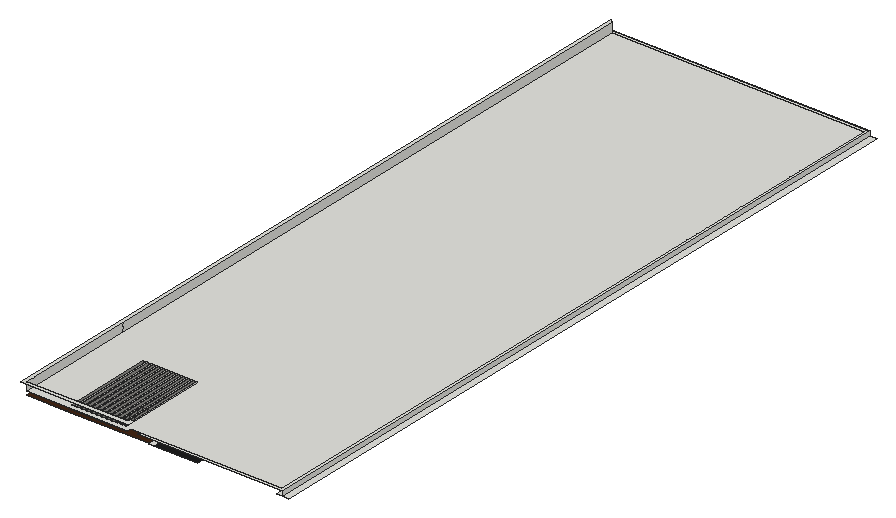
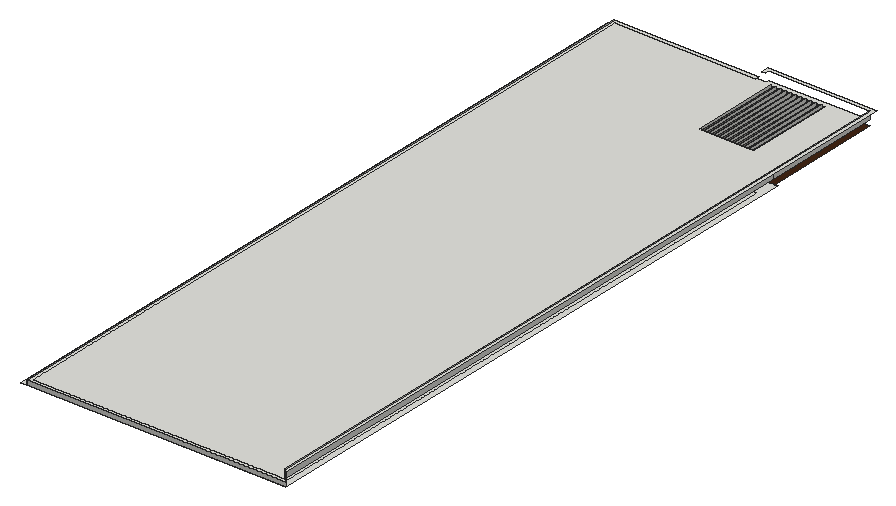
# SketchUp Ruby script. Lengths in inches.
U = 1.inch
M = Sketchup.active_model
def pt(a) = Geom::Point3d.new(a.map { |v| v * U })
def face(e, loops, mat)
  f = e.add_face(loops[0].map { |a| pt(a) })
  loops[1..].each { |l| e.add_face(l.map { |a| pt(a) }).erase! }
  f.material = f.back_material = mat if mat
  f
end
# faces: each face lists its corners as indices into pts; further lists are holes
def faces(e, pts, list, mat = nil) = list.each { |f| face(e, (f[0].is_a?(Array) ? f : [f]).map { |l| l.map { |i| pts[i] } }, mat) }
# xy, xz, yz: faces in a plane at the given z, y or x. An outline is a flat list of corners, or four numbers for a rectangle; further outlines are holes
def ring(l) = l.size == 4 ? [[l[0], l[1]], [l[2], l[1]], [l[2], l[3]], [l[0], l[3]]] : l.each_slice(2).to_a
def flat(e, list, mat, &to3) = list.each { |f| face(e, (f[0].is_a?(Array) ? f : [f]).map { |l| ring(l).map { |u, v| to3.(u, v) } }, mat) }
def xy(e, z, list, mat = nil) = flat(e, list, mat) { |x, y| [x, y, z] }
def xz(e, y, list, mat = nil) = flat(e, list, mat) { |x, z| [x, y, z] }
def yz(e, x, list, mat = nil) = flat(e, list, mat) { |y, z| [x, y, z] }
def lines(e, pts, list) = list.each { |a, b| e.add_line(pt(pts[a]), pt(pts[b])) }
# prism: a flat outline (further loops are holes) pulled along v
def prism(e, loops, v, mat = nil)
  f = face(e, loops, mat); d = Geom::Vector3d.new(v.map { |x| x * U })
  f.pushpull(f.normal.samedirection?(d) ? d.length : -d.length)
end
def box(e, o, s, mat = nil) = prism(e, [[o, [o[0] + s[0], o[1], o[2]], [o[0] + s[0], o[1] + s[1], o[2]], [o[0], o[1] + s[1], o[2]]]], [0, 0, s[2]], mat)
def at(x, y, z, deg = 0) = Geom::Transformation.translation(pt([x, y, z])) * Geom::Transformation.rotation(ORIGIN, Z_AXIS, deg.degrees)
def axes(o, x, y, z) = Geom::Transformation.new([*x, 0, *y, 0, *z, 0, *pt(o).to_a, 1])
def part(name) = M.definitions.add(name)
# library, detail: a bought-in or finely detailed component or shape, given as its bounding box
def library(name, o, s) = part(name).tap { |d| box(d.entities, o, s) }
def detail(e, o, s) = box(e.add_group.entities, o, s)
def put(e, d, t, mat = nil) = e.add_instance(d, t).tap { |i| i.material = mat if mat }
def group(e, t, mat = nil) = e.add_group.tap { |g| g.transformation = t; g.material = mat if mat }.entities
root = M.entities
M.materials.add("[Color M08]").color = [30, 30, 30]
M.materials.add("[Field Square Tile]").color = [211, 167, 108]
M.materials.add("[Granite Light Gray]").color = [149, 148, 144]
M.materials.add("[Wood Veneer 01]").color = [66, 38, 20]
xy(root,380.5,[[1555.29,511.08,1555.29,1825.82,1107.53,1825.82,1107.53,762.17,1323.53,762.17,1323.53,727.2,1097.72,727.2,1097.72,1835.625,1565.1,1835.625,1565.1,511.08],[1323.53,511.08,1332.45,589.83],[1565.1,511.08,1576.91,1835.625],[1323.53,589.83,1323.53,762.17,1107.53,762.17,1107.53,1825.82,1555.29,1825.82,1555.29,589.83,1508.52,589.83,1508.52,697.21,1413.21,697.21,1413.21,738.02,1332.45,738.02,1332.45,697.21,1323.83,697.21,1323.83,589.83],[1323.83,589.83,1332.45,697.21],
  [1413.21,589.83,1508.52,697.21],[1332.45,697.21,1413.21,738.02]])
xy(root,380.5,[[1332.45,511.08,1413.21,697.21]],"[Color M08]")
xy(root,380.5,[[[1102.55,512.27,1174.48,727.2],[1119.58,606.01,1121.1,606.38,1122.48,607.14,1123.61,608.22,1124.42,609.56,1124.85,611.0625,1124.89,612.63,1124.51,614.15,1123.76,615.52,1122.67,616.65,1121.33,617.46,1119.83,617.9,1118.26,617.93,1116.74,617.56,1115.37,616.81,1114.24,615.72,1113.43,614.38,1112.99,612.875,1112.96,611.3125,1113.33,609.79,1114.09,608.42,1115.17,607.29,1116.51,606.48,1118.02,606.04],[1119.58,554.26,1121.1,554.63,1122.48,555.39,1123.61,556.47,1124.42,557.81,1124.85,559.3125,1124.89,560.88,1124.51,562.4,1123.76,563.77,1122.67,564.9,1121.33,565.71,1119.83,566.15,1118.26,566.18,1116.74,565.81,1115.37,565.06,1114.24,563.97,1113.43,562.63,1112.99,561.125,1112.96,559.5625,1113.33,558.04,1114.09,556.67,1115.17,555.54,1116.51,554.73,1118.02,554.29],[1119.58,523.51,1121.1,523.88,1122.48,524.64,1123.61,525.72,1124.42,527.06,1124.85,528.5625,1124.89,530.13,1124.51,531.65,1123.76,533.02,1122.67,534.15,1121.33,534.96,1119.83,535.4,1118.26,535.43,1116.74,535.06,1115.37,534.31,1114.24,533.22,1113.43,531.88,1112.99,530.375,1112.96,528.8125,1113.33,527.29,1114.09,525.92,1115.17,524.79,1116.51,523.98,1118.02,523.54],[1119.58,666.01,1121.1,666.38,1122.48,667.14,1123.61,668.22,1124.42,669.56,1124.85,671.0625,1124.89,672.63,1124.51,674.15,1123.76,675.52,1122.67,676.65,1121.33,677.46,1119.83,677.9,1118.26,677.93,1116.74,677.56,1115.37,676.81,1114.24,675.72,1113.43,674.38,1112.99,672.875,1112.96,671.3125,1113.33,669.79,1114.09,668.42,1115.17,667.29,1116.51,666.48,1118.02,666.04],[1159.33,606.01,1160.85,606.38,1162.23,607.14,1163.36,608.22,1164.17,609.56,1164.6,611.0625,1164.64,612.63,1164.26,614.15,1163.51,615.52,1162.42,616.65,1161.08,617.46,1159.58,617.9,1158.01,617.93,1156.49,617.56,1155.12,616.81,1153.99,615.72,1153.18,614.38,1152.74,612.875,1152.71,611.3125,1153.08,609.79,1153.84,608.42,1154.92,607.29,1156.26,606.48,1157.77,606.04],[1159.33,554.26,1160.85,554.63,1162.23,555.39,1163.36,556.47,1164.17,557.81,1164.6,559.3125,1164.64,560.88,1164.26,562.4,1163.51,563.77,1162.42,564.9,1161.08,565.71,1159.58,566.15,1158.01,566.18,1156.49,565.81,1155.12,565.06,1153.99,563.97,1153.18,562.63,1152.74,561.125,1152.71,559.5625,1153.08,558.04,1153.84,556.67,1154.92,555.54,1156.26,554.73,1157.77,554.29],[1159.33,523.51,1160.85,523.88,1162.23,524.64,1163.36,525.72,1164.17,527.06,1164.6,528.5625,1164.64,530.13,1164.26,531.65,1163.51,533.02,1162.42,534.15,1161.08,534.96,1159.58,535.4,1158.01,535.43,1156.49,535.06,1155.12,534.31,1153.99,533.22,1153.18,531.88,1152.74,530.375,1152.71,528.8125,1153.08,527.29,1153.84,525.92,1154.92,524.79,1156.26,523.98,1157.77,523.54],[1159.33,666.01,1160.85,666.38,1162.23,667.14,1163.36,668.22,1164.17,669.56,1164.6,671.0625,1164.64,672.63,1164.26,674.15,1163.51,675.52,1162.42,676.65,1161.08,677.46,1159.58,677.9,1158.01,677.93,1156.49,677.56,1155.12,676.81,1153.99,675.72,1153.18,674.38,1152.74,672.875,1152.71,671.3125,1153.08,669.79,1153.84,668.42,1154.92,667.29,1156.26,666.48,1157.77,666.04]],[[1174.48,512.27,1323.53,727.2],[1269.93,519.43,1276.18,680.49],[1260.81,519.43,1267.06,680.49],[1251.68,519.43,1257.93,680.49],[1242.56,519.43,1248.81,680.49],[1233.43,519.43,1239.68,680.49],[1224.31,519.43,1230.56,680.49],[1215.18,519.43,1221.43,680.49],[1206.06,519.43,1212.31,680.49],[1196.93,519.43,1203.18,680.49],[1187.81,519.43,1194.06,680.49],[1178.68,519.43,1184.93,680.49]]],"[Wood Veneer 01]")
xy(root,381.875,[[1119.58,554.26,1118.02,554.29,1116.51,554.73,1115.17,555.54,1114.09,556.67,1113.33,558.04,1112.96,559.5625,1112.99,561.125,1113.43,562.63,1114.24,563.97,1115.37,565.06,1116.74,565.81,1118.26,566.18,1119.83,566.15,1121.33,565.71,1122.67,564.9,1123.76,563.77,1124.51,562.4,1124.89,560.88,1124.85,559.3125,1124.42,557.81,1123.61,556.47,1122.48,555.39,1121.1,554.63],[1159.33,554.26,1157.77,554.29,1156.26,554.73,1154.92,555.54,1153.84,556.67,1153.08,558.04,1152.71,559.5625,1152.74,561.125,1153.18,562.63,1153.99,563.97,1155.12,565.06,1156.49,565.81,1158.01,566.18,1159.58,566.15,1161.08,565.71,1162.42,564.9,1163.51,563.77,1164.26,562.4,1164.64,560.88,1164.6,559.3125,1164.17,557.81,1163.36,556.47,1162.23,555.39,1160.85,554.63],[1119.58,606.01,1118.02,606.04,1116.51,606.48,1115.17,607.29,1114.09,608.42,1113.33,609.79,1112.96,611.3125,1112.99,612.875,1113.43,614.38,1114.24,615.72,1115.37,616.81,1116.74,617.56,1118.26,617.93,1119.83,617.9,1121.33,617.46,1122.67,616.65,1123.76,615.52,1124.51,614.15,1124.89,612.63,1124.85,611.0625,1124.42,609.56,1123.61,608.22,1122.48,607.14,1121.1,606.38],[1159.33,606.01,1157.77,606.04,1156.26,606.48,1154.92,607.29,1153.84,608.42,1153.08,609.79,1152.71,611.3125,1152.74,612.875,1153.18,614.38,1153.99,615.72,1155.12,616.81,1156.49,617.56,1158.01,617.93,1159.58,617.9,1161.08,617.46,1162.42,616.65,1163.51,615.52,1164.26,614.15,1164.64,612.63,1164.6,611.0625,1164.17,609.56,1163.36,608.22,1162.23,607.14,1160.85,606.38],[1119.58,666.01,1118.02,666.04,1116.51,666.48,1115.17,667.29,1114.09,668.42,1113.33,669.79,1112.96,671.3125,1112.99,672.875,1113.43,674.38,1114.24,675.72,1115.37,676.81,1116.74,677.56,1118.26,677.93,1119.83,677.9,1121.33,677.46,1122.67,676.65,1123.76,675.52,1124.51,674.15,1124.89,672.63,1124.85,671.0625,1124.42,669.56,1123.61,668.22,1122.48,667.14,1121.1,666.38],
  [1159.33,666.01,1157.77,666.04,1156.26,666.48,1154.92,667.29,1153.84,668.42,1153.08,669.79,1152.71,671.3125,1152.74,672.875,1153.18,674.38,1153.99,675.72,1155.12,676.81,1156.49,677.56,1158.01,677.93,1159.58,677.9,1161.08,677.46,1162.42,676.65,1163.51,675.52,1164.26,674.15,1164.64,672.63,1164.6,671.0625,1164.17,669.56,1163.36,668.22,1162.23,667.14,1160.85,666.38]],"[Field Square Tile]")
xy(root,388.625,[[[1104.06,510.87,1287.38,510.87,1287.38,517.43,1558.75,517.43,1558.75,1829.28,1104.06,1829.28],[1178.68,519.43,1184.93,680.49],[1187.81,519.43,1194.06,680.49],[1196.93,519.43,1203.18,680.49],[1206.06,519.43,1212.31,680.49],[1215.18,519.43,1221.43,680.49],[1224.31,519.43,1230.56,680.49],[1233.43,519.43,1239.68,680.49],[1242.56,519.43,1248.81,680.49],[1251.68,519.43,1257.93,680.49],[1260.81,519.43,1267.06,680.49],[1269.93,519.43,1276.18,680.49]],[1304.4375,511.08,1565.1,511.08,1565.1,1835.625,1097.72,1835.625,1104.06,1829.28,1558.75,1829.28,1558.75,517.43,1304.4375,517.43]])
xy(root,403.8125,[[1097.72,504.52,1293.73,504.52,1293.73,517.43,1287.38,517.43,1287.38,510.87,1104.06,510.87,1104.06,1829.28,1097.72,1835.625]])
xz(root,680.49,[[1178.68,380.5,1184.93,388.625],[1187.81,380.5,1194.06,388.625],[1196.93,380.5,1203.18,388.625],[1206.06,380.5,1212.31,388.625],[1215.18,380.5,1221.43,388.625],
  [1224.31,380.5,1230.56,388.625],[1233.43,380.5,1239.68,388.625],[1242.56,380.5,1248.81,388.625],[1251.68,380.5,1257.93,388.625],[1260.81,380.5,1267.06,388.625],
  [1269.93,380.5,1276.18,388.625]],"[Granite Light Gray]")
xz(root,1835.625,[[1097.72,380.5,1565.1,388.625]])
yz(root,1104.06,[[510.87,388.625,727.2,403.8125],[727.2,388.625,1829.28,403.8125]])
yz(root,1178.68,[[519.43,380.5,680.49,388.625]],"[Granite Light Gray]")
yz(root,1184.93,[[519.43,380.5,680.49,388.625]])
yz(root,1187.81,[[519.43,380.5,680.49,388.625]],"[Granite Light Gray]")
yz(root,1194.06,[[519.43,380.5,680.49,388.625]])
yz(root,1196.93,[[519.43,380.5,680.49,388.625]],"[Granite Light Gray]")
yz(root,1203.18,[[519.43,380.5,680.49,388.625]])
yz(root,1206.06,[[519.43,380.5,680.49,388.625]],"[Granite Light Gray]")
yz(root,1212.31,[[519.43,380.5,680.49,388.625]])
yz(root,1215.18,[[519.43,380.5,680.49,388.625]],"[Granite Light Gray]")
yz(root,1221.43,[[519.43,380.5,680.49,388.625]])
yz(root,1224.31,[[519.43,380.5,680.49,388.625]],"[Granite Light Gray]")
yz(root,1230.56,[[519.43,380.5,680.49,388.625]])
yz(root,1233.43,[[519.43,380.5,680.49,388.625]],"[Granite Light Gray]")
yz(root,1239.68,[[519.43,380.5,680.49,388.625]])
yz(root,1242.56,[[519.43,380.5,680.49,388.625]],"[Granite Light Gray]")
yz(root,1248.81,[[519.43,380.5,680.49,388.625]])
yz(root,1251.68,[[519.43,380.5,680.49,388.625]],"[Granite Light Gray]")
yz(root,1257.93,[[519.43,380.5,680.49,388.625]])
yz(root,1260.81,[[519.43,380.5,680.49,388.625]],"[Granite Light Gray]")
yz(root,1267.06,[[519.43,380.5,680.49,388.625]])
yz(root,1269.93,[[519.43,380.5,680.49,388.625]],"[Granite Light Gray]")
yz(root,1276.18,[[519.43,380.5,680.49,388.625]])
yz(root,1565.1,[[511.08,380.5,1835.625,388.625]])
p = [[1118.26,535.43,380.5],[1119.83,535.4,380.5],[1119.83,535.4,381.875],[1118.26,535.43,381.875],[1158.01,535.43,380.5],[1159.58,535.4,380.5],
  [1159.58,535.4,381.875],[1158.01,535.43,381.875],[1118.02,554.29,380.5],[1116.51,554.73,380.5],[1116.51,554.73,381.875],[1118.02,554.29,381.875],
  [1119.58,554.26,380.5],[1119.58,554.26,381.875],[1121.1,554.63,380.5],[1121.1,554.63,381.875],[1157.77,554.29,380.5],[1156.26,554.73,380.5],
  [1156.26,554.73,381.875],[1157.77,554.29,381.875],[1159.33,554.26,380.5],[1159.33,554.26,381.875],[1160.85,554.63,380.5],[1160.85,554.63,381.875],
  [1122.48,555.39,380.5],[1122.48,555.39,381.875],[1162.23,555.39,380.5],[1162.23,555.39,381.875],[1115.17,555.54,380.5],[1115.17,555.54,381.875],
  [1154.92,555.54,380.5],[1154.92,555.54,381.875],[1123.61,556.47,380.5],[1123.61,556.47,381.875],[1163.36,556.47,380.5],[1163.36,556.47,381.875],
  [1114.09,556.67,380.5],[1114.09,556.67,381.875],[1153.84,556.67,380.5],[1153.84,556.67,381.875],[1124.42,557.81,380.5],[1124.42,557.81,381.875],
  [1164.17,557.81,380.5],[1164.17,557.81,381.875],[1113.33,558.04,380.5],[1113.33,558.04,381.875],[1153.08,558.04,380.5],[1153.08,558.04,381.875],
  [1124.85,559.3125,380.5],[1124.85,559.3125,381.875],[1164.6,559.3125,380.5],[1164.6,559.3125,381.875],[1112.96,559.5625,380.5],[1112.96,559.5625,381.875],
  [1152.71,559.5625,380.5],[1152.71,559.5625,381.875],[1124.89,560.88,380.5],[1124.89,560.88,381.875],[1164.64,560.88,380.5],[1164.64,560.88,381.875],
  [1112.99,561.125,380.5],[1112.99,561.125,381.875],[1152.74,561.125,380.5],[1152.74,561.125,381.875],[1124.51,562.4,380.5],[1124.51,562.4,381.875],
  [1164.26,562.4,380.5],[1164.26,562.4,381.875],[1113.43,562.63,380.5],[1113.43,562.63,381.875],[1153.18,562.63,380.5],[1153.18,562.63,381.875],
  [1123.76,563.77,380.5],[1123.76,563.77,381.875],[1163.51,563.77,380.5],[1163.51,563.77,381.875],[1114.24,563.97,380.5],[1114.24,563.97,381.875],
  [1153.99,563.97,380.5],[1153.99,563.97,381.875],[1122.67,564.9,380.5],[1122.67,564.9,381.875],[1162.42,564.9,380.5],[1162.42,564.9,381.875],
  [1115.37,565.06,380.5],[1115.37,565.06,381.875],[1155.12,565.06,380.5],[1155.12,565.06,381.875],[1121.33,565.71,380.5],[1121.33,565.71,381.875],
  [1161.08,565.71,380.5],[1161.08,565.71,381.875],[1116.74,565.81,380.5],[1116.74,565.81,381.875],[1156.49,565.81,380.5],[1156.49,565.81,381.875],
  [1119.83,566.15,380.5],[1119.83,566.15,381.875],[1159.58,566.15,380.5],[1159.58,566.15,381.875],[1118.26,566.18,380.5],[1118.26,566.18,381.875],
  [1158.01,566.18,380.5],[1158.01,566.18,381.875],[1118.02,606.04,380.5],[1116.51,606.48,380.5],[1116.51,606.48,381.875],[1118.02,606.04,381.875],
  [1119.58,606.01,380.5],[1119.58,606.01,381.875],[1121.1,606.38,380.5],[1121.1,606.38,381.875],[1157.77,606.04,380.5],[1156.26,606.48,380.5],
  [1156.26,606.48,381.875],[1157.77,606.04,381.875],[1159.33,606.01,380.5],[1159.33,606.01,381.875],[1160.85,606.38,380.5],[1160.85,606.38,381.875],
  [1122.48,607.14,380.5],[1122.48,607.14,381.875],[1162.23,607.14,380.5],[1162.23,607.14,381.875],[1115.17,607.29,380.5],[1115.17,607.29,381.875],
  [1154.92,607.29,380.5],[1154.92,607.29,381.875],[1123.61,608.22,380.5],[1123.61,608.22,381.875],[1163.36,608.22,380.5],[1163.36,608.22,381.875],
  [1114.09,608.42,380.5],[1114.09,608.42,381.875],[1153.84,608.42,380.5],[1153.84,608.42,381.875],[1124.42,609.56,380.5],[1124.42,609.56,381.875],
  [1164.17,609.56,380.5],[1164.17,609.56,381.875],[1113.33,609.79,380.5],[1113.33,609.79,381.875],[1153.08,609.79,380.5],[1153.08,609.79,381.875],
  [1124.85,611.0625,380.5],[1124.85,611.0625,381.875],[1164.6,611.0625,380.5],[1164.6,611.0625,381.875],[1112.96,611.3125,380.5],[1112.96,611.3125,381.875],
  [1152.71,611.3125,380.5],[1152.71,611.3125,381.875],[1124.89,612.63,380.5],[1124.89,612.63,381.875],[1164.64,612.63,380.5],[1164.64,612.63,381.875],
  [1112.99,612.875,380.5],[1112.99,612.875,381.875],[1152.74,612.875,380.5],[1152.74,612.875,381.875],[1124.51,614.15,380.5],[1124.51,614.15,381.875],
  [1164.26,614.15,380.5],[1164.26,614.15,381.875],[1113.43,614.38,380.5],[1113.43,614.38,381.875],[1153.18,614.38,380.5],[1153.18,614.38,381.875],
  [1123.76,615.52,380.5],[1123.76,615.52,381.875],[1163.51,615.52,380.5],[1163.51,615.52,381.875],[1114.24,615.72,380.5],[1114.24,615.72,381.875],
  [1153.99,615.72,380.5],[1153.99,615.72,381.875],[1122.67,616.65,380.5],[1122.67,616.65,381.875],[1162.42,616.65,380.5],[1162.42,616.65,381.875],
  [1115.37,616.81,380.5],[1115.37,616.81,381.875],[1155.12,616.81,380.5],[1155.12,616.81,381.875],[1121.33,617.46,380.5],[1121.33,617.46,381.875],
  [1161.08,617.46,380.5],[1161.08,617.46,381.875],[1116.74,617.56,380.5],[1116.74,617.56,381.875],[1156.49,617.56,380.5],[1156.49,617.56,381.875],
  [1119.83,617.9,380.5],[1119.83,617.9,381.875],[1159.58,617.9,380.5],[1159.58,617.9,381.875],[1118.26,617.93,380.5],[1118.26,617.93,381.875],
  [1158.01,617.93,380.5],[1158.01,617.93,381.875],[1118.02,666.04,380.5],[1116.51,666.48,380.5],[1116.51,666.48,381.875],[1118.02,666.04,381.875],
  [1119.58,666.01,380.5],[1119.58,666.01,381.875],[1121.1,666.38,380.5],[1121.1,666.38,381.875],[1157.77,666.04,380.5],[1156.26,666.48,380.5],
  [1156.26,666.48,381.875],[1157.77,666.04,381.875],[1159.33,666.01,380.5],[1159.33,666.01,381.875],[1160.85,666.38,380.5],[1160.85,666.38,381.875],
  [1122.48,667.14,380.5],[1122.48,667.14,381.875],[1162.23,667.14,380.5],[1162.23,667.14,381.875],[1115.17,667.29,380.5],[1115.17,667.29,381.875],
  [1154.92,667.29,380.5],[1154.92,667.29,381.875],[1123.61,668.22,380.5],[1123.61,668.22,381.875],[1163.36,668.22,380.5],[1163.36,668.22,381.875],
  [1114.09,668.42,380.5],[1114.09,668.42,381.875],[1153.84,668.42,380.5],[1153.84,668.42,381.875],[1124.42,669.56,380.5],[1124.42,669.56,381.875],
  [1164.17,669.56,380.5],[1164.17,669.56,381.875],[1113.33,669.79,380.5],[1113.33,669.79,381.875],[1153.08,669.79,380.5],[1153.08,669.79,381.875],
  [1124.85,671.0625,380.5],[1124.85,671.0625,381.875],[1164.6,671.0625,380.5],[1164.6,671.0625,381.875],[1112.96,671.3125,380.5],[1112.96,671.3125,381.875],
  [1152.71,671.3125,380.5],[1152.71,671.3125,381.875],[1124.89,672.63,380.5],[1124.89,672.63,381.875],[1164.64,672.63,380.5],[1164.64,672.63,381.875],
  [1112.99,672.875,380.5],[1112.99,672.875,381.875],[1152.74,672.875,380.5],[1152.74,672.875,381.875],[1124.51,674.15,380.5],[1124.51,674.15,381.875],
  [1164.26,674.15,380.5],[1164.26,674.15,381.875],[1113.43,674.38,380.5],[1113.43,674.38,381.875],[1153.18,674.38,380.5],[1153.18,674.38,381.875],
  [1123.76,675.52,380.5],[1123.76,675.52,381.875],[1163.51,675.52,380.5],[1163.51,675.52,381.875],[1114.24,675.72,380.5],[1114.24,675.72,381.875],
  [1153.99,675.72,380.5],[1153.99,675.72,381.875],[1122.67,676.65,380.5],[1122.67,676.65,381.875],[1162.42,676.65,380.5],[1162.42,676.65,381.875],
  [1115.37,676.81,380.5],[1115.37,676.81,381.875],[1155.12,676.81,380.5],[1155.12,676.81,381.875],[1121.33,677.46,380.5],[1121.33,677.46,381.875],
  [1161.08,677.46,380.5],[1161.08,677.46,381.875],[1116.74,677.56,380.5],[1116.74,677.56,381.875],[1156.49,677.56,380.5],[1156.49,677.56,381.875],
  [1119.83,677.9,380.5],[1119.83,677.9,381.875],[1159.58,677.9,380.5],[1159.58,677.9,381.875],[1118.26,677.93,380.5],[1118.26,677.93,381.875],
  [1158.01,677.93,380.5],[1158.01,677.93,381.875],[1104.06,1829.28,388.625],[1097.72,1835.625,388.625],[1097.72,1835.625,403.8125],[1104.06,1829.28,403.8125]]
faces(root,p,[[0,1,2,3],[4,5,6,7],[8,9,10,11],[12,8,11,13],[14,12,13,15],[16,17,18,19],[20,16,19,21],[22,20,21,23],
  [24,14,15,25],[26,22,23,27],[9,28,29,10],[17,30,31,18],[32,24,25,33],[34,26,27,35],[28,36,37,29],[30,38,39,31],
  [40,32,33,41],[42,34,35,43],[36,44,45,37],[38,46,47,39],[48,40,41,49],[50,42,43,51],[44,52,53,45],[46,54,55,47],
  [56,48,49,57],[58,50,51,59],[52,60,61,53],[54,62,63,55],[64,56,57,65],[66,58,59,67],[60,68,69,61],[62,70,71,63],
  [72,64,65,73],[74,66,67,75],[68,76,77,69],[70,78,79,71],[80,72,73,81],[82,74,75,83],[76,84,85,77],[78,86,87,79],
  [88,80,81,89],[90,82,83,91],[84,92,93,85],[86,94,95,87],[96,88,89,97],[98,90,91,99],[92,100,101,93],[94,102,103,95],
  [100,96,97,101],[102,98,99,103],[104,105,106,107],[108,104,107,109],[110,108,109,111],[112,113,114,115],[116,112,115,117],[118,116,117,119],
  [120,110,111,121],[122,118,119,123],[105,124,125,106],[113,126,127,114],[128,120,121,129],[130,122,123,131],[124,132,133,125],[126,134,135,127],
  [136,128,129,137],[138,130,131,139],[132,140,141,133],[134,142,143,135],[144,136,137,145],[146,138,139,147],[140,148,149,141],[142,150,151,143],
  [152,144,145,153],[154,146,147,155],[148,156,157,149],[150,158,159,151],[160,152,153,161],[162,154,155,163],[156,164,165,157],[158,166,167,159],
  [168,160,161,169],[170,162,163,171],[164,172,173,165],[166,174,175,167],[176,168,169,177],[178,170,171,179],[172,180,181,173],[174,182,183,175],
  [184,176,177,185],[186,178,179,187],[180,188,189,181],[182,190,191,183],[192,184,185,193],[194,186,187,195],[188,196,197,189],[190,198,199,191],
  [196,192,193,197],[198,194,195,199],[200,201,202,203],[204,200,203,205],[206,204,205,207],[208,209,210,211],[212,208,211,213],[214,212,213,215],
  [216,206,207,217],[218,214,215,219],[201,220,221,202],[209,222,223,210],[224,216,217,225],[226,218,219,227],[220,228,229,221],[222,230,231,223],
  [232,224,225,233],[234,226,227,235],[228,236,237,229],[230,238,239,231],[240,232,233,241],[242,234,235,243],[236,244,245,237],[238,246,247,239],
  [248,240,241,249],[250,242,243,251],[244,252,253,245],[246,254,255,247],[256,248,249,257],[258,250,251,259],[252,260,261,253],[254,262,263,255],
  [264,256,257,265],[266,258,259,267],[260,268,269,261],[262,270,271,263],[272,264,265,273],[274,266,267,275],[268,276,277,269],[270,278,279,271],
  [280,272,273,281],[282,274,275,283],[276,284,285,277],[278,286,287,279],[288,280,281,289],[290,282,283,291],[284,292,293,285],[286,294,295,287],
  [292,288,289,293],[294,290,291,295]],"[Field Square Tile]")
faces(root,p,[[296,297,298,299]])
